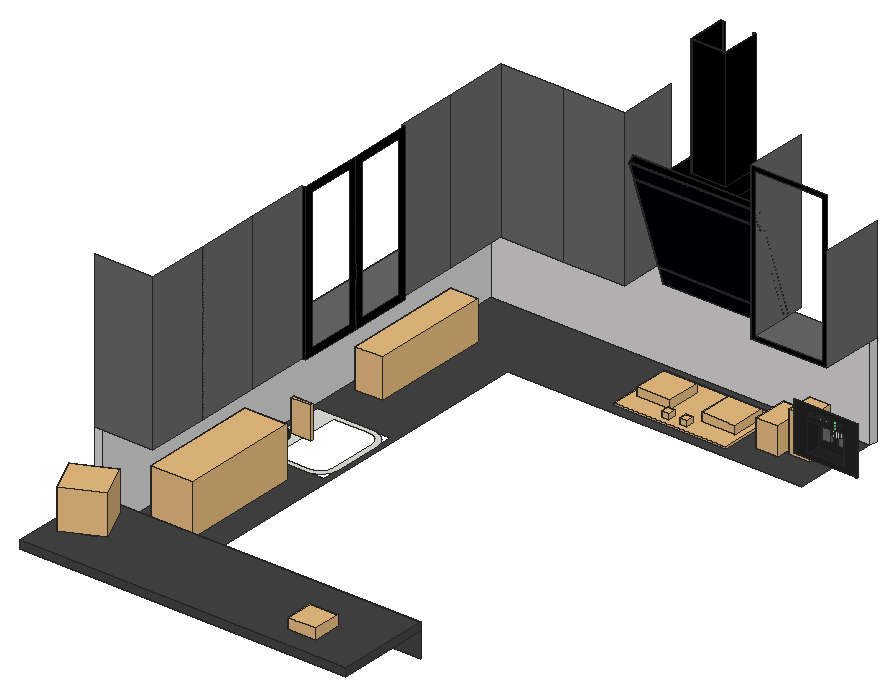
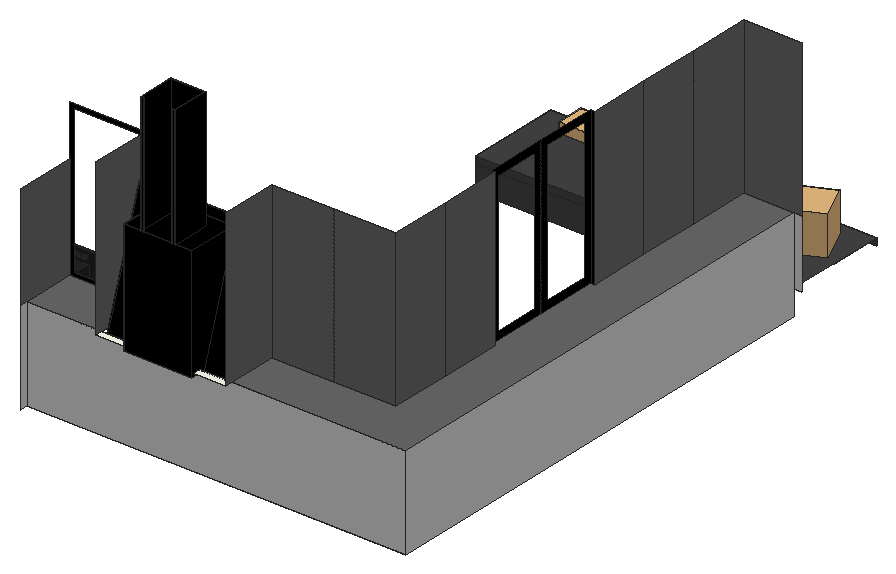
# SketchUp Ruby script. Lengths in inches.
U = 1.inch
M = Sketchup.active_model
def pt(a) = Geom::Point3d.new(a.map { |v| v * U })
def face(e, loops, mat)
  f = e.add_face(loops[0].map { |a| pt(a) })
  loops[1..].each { |l| e.add_face(l.map { |a| pt(a) }).erase! }
  f.material = f.back_material = mat if mat
  f
end
# faces: each face lists its corners as indices into pts; further lists are holes
def faces(e, pts, list, mat = nil) = list.each { |f| face(e, (f[0].is_a?(Array) ? f : [f]).map { |l| l.map { |i| pts[i] } }, mat) }
# xy, xz, yz: faces in a plane at the given z, y or x. An outline is a flat list of corners, or four numbers for a rectangle; further outlines are holes
def ring(l) = l.size == 4 ? [[l[0], l[1]], [l[2], l[1]], [l[2], l[3]], [l[0], l[3]]] : l.each_slice(2).to_a
def flat(e, list, mat, &to3) = list.each { |f| face(e, (f[0].is_a?(Array) ? f : [f]).map { |l| ring(l).map { |u, v| to3.(u, v) } }, mat) }
def xy(e, z, list, mat = nil) = flat(e, list, mat) { |x, y| [x, y, z] }
def xz(e, y, list, mat = nil) = flat(e, list, mat) { |x, z| [x, y, z] }
def yz(e, x, list, mat = nil) = flat(e, list, mat) { |y, z| [x, y, z] }
def lines(e, pts, list) = list.each { |a, b| e.add_line(pt(pts[a]), pt(pts[b])) }
# prism: a flat outline (further loops are holes) pulled along v
def prism(e, loops, v, mat = nil)
  f = face(e, loops, mat); d = Geom::Vector3d.new(v.map { |x| x * U })
  f.pushpull(f.normal.samedirection?(d) ? d.length : -d.length)
end
def box(e, o, s, mat = nil) = prism(e, [[o, [o[0] + s[0], o[1], o[2]], [o[0] + s[0], o[1] + s[1], o[2]], [o[0], o[1] + s[1], o[2]]]], [0, 0, s[2]], mat)
def at(x, y, z, deg = 0) = Geom::Transformation.translation(pt([x, y, z])) * Geom::Transformation.rotation(ORIGIN, Z_AXIS, deg.degrees)
def axes(o, x, y, z) = Geom::Transformation.new([*x, 0, *y, 0, *z, 0, *pt(o).to_a, 1])
def part(name) = M.definitions.add(name)
# library, detail: a bought-in or finely detailed component or shape, given as its bounding box
def library(name, o, s) = part(name).tap { |d| box(d.entities, o, s) }
def detail(e, o, s) = box(e.add_group.entities, o, s)
def put(e, d, t, mat = nil) = e.add_instance(d, t).tap { |i| i.material = mat if mat }
def group(e, t, mat = nil) = e.add_group.tap { |g| g.transformation = t; g.material = mat if mat }.entities
root = M.entities
M.materials.add("78970012").color = [84, 74, 27]
M.materials.add("Brush Stainles Steel").color = [21, 26, 31]
M.materials.add("Material60").color = [0, 0, 8]
M.materials.add("[0046_Gold]").color = [255, 215, 0]
M.materials.add("[0053_Ivory]").color = [255, 255, 240]
M.materials.add("[0067_PaleGreen]").color = [152, 251, 152]
M.materials.add("[0070_SpringGreen]").color = [0, 255, 127]
M.materials.add("[0072_DarkSeaGreen]").color = [143, 188, 143]
M.materials.add("[0087_Cyan]").color = [0, 255, 255]
M.materials.add("[0088_Aquamarine]").color = [127, 255, 212]
M.materials.add("[0096_SkyBlue]").color = [135, 206, 235]
M.materials.add("[0117_GhostWhite]").color = [248, 248, 255]
M.materials.add("[0131_Silver]").color = [192, 192, 192]
M.materials.add("[0134_DimGray]").color = [105, 105, 105]
M.materials.add("[0136_Charcoal]").color = [35, 35, 35]
M.materials.add("[0137_Black]").color = [0, 0, 0]
M.materials.add("[Granite Dark Gray]").color = [69, 68, 68]
M.materials.add("[Stone Vein Gray]").color = [219, 217, 217]
M.materials.add("stainless-steel2").color = [0, 0, 0]
c1 = library("Group70\#2",[-9.87,-9.87,-55.07],[19.74,112.51,110.23])
c2 = library("组\#1",[0,0,0],[5.3125,6.7,10.38])
c3 = library("Gas burner",[0,0.01,0],[8.66,8.66,2.72])
c4 = part("Bathroom Tap Knob")
xy(c4.entities,1.57,[[0.59,0,0.74,0.02,0.89,0.08,1.01,0.17,1.1,0.3,1.16,0.4375,1.18,0.59,1.16,0.74,1.1,0.89,1.01,1.01,0.89,1.1,0.74,1.16,0.59,1.18,0.4375,1.16,0.3,1.1,0.17,1.01,0.08,0.89,0.02,0.74,0,0.59,0.02,0.4375,0.08,0.3,0.17,0.17,0.3,0.08,0.4375,0.02]])
p = [[0.3,0.08,0],[0.4375,0.02,0],[0.4375,0.02,1.57],[0.3,0.08,1.57],[0.59,0,0],[0.59,0,1.57],
  [0.74,0.02,0],[0.74,0.02,1.57],[0.89,0.08,0],[0.89,0.08,1.57],[0.17,0.17,0],[0.17,0.17,1.57],
  [1.01,0.17,0],[1.01,0.17,1.57],[0.08,0.3,0],[0.08,0.3,1.57],[1.1,0.3,0],[1.1,0.3,1.57],
  [0.02,0.4375,0],[0.02,0.4375,1.57],[1.16,0.4375,0],[1.16,0.4375,1.57],[0,0.59,0],[0,0.59,1.57],
  [1.18,0.59,0],[1.18,0.59,1.57],[0.02,0.74,0],[0.02,0.74,1.57],[1.16,0.74,0],[1.16,0.74,1.57],
  [0.08,0.89,0],[0.08,0.89,1.57],[1.1,0.89,0],[1.1,0.89,1.57],[0.17,1.01,0],[0.17,1.01,1.57],
  [1.01,1.01,0],[1.01,1.01,1.57],[0.3,1.1,0],[0.3,1.1,1.57],[0.89,1.1,0],[0.89,1.1,1.57],
  [0.4375,1.16,0],[0.4375,1.16,1.57],[0.74,1.16,0],[0.74,1.16,1.57],[0.59,1.18,0],[0.59,1.18,1.57]]
faces(c4.entities,p,[[0,1,2,3],[1,4,5,2],[4,6,7,5],[6,8,9,7],[10,0,3,11],[8,12,13,9],[14,10,11,15],[12,16,17,13],
  [18,14,15,19],[16,20,21,17],[22,18,19,23],[20,24,25,21],[26,22,23,27],[24,28,29,25],[30,26,27,31],[28,32,33,29],
  [34,30,31,35],[32,36,37,33],[38,34,35,39],[36,40,41,37],[42,38,39,43],[40,44,45,41],[46,42,43,47],[44,46,47,45]])
c5 = library("Bathroom Tap",[0,0,0],[4.72,0.79,8.27])
c6 = library("Group\#260",[0,0,0],[30.82,7.02,10])
c7 = library("GasStove_E",[0,-1.18,0],[28.74,16.53,0.59])
c8 = library("knifes set",[0,0,0],[30.4,10.88,12.79])
c9 = library("Group71\#2",[-14.38,-9.9375,-11.98],[31.13,19.875,24.75])
c10 = library("Burner control knob",[0,0,0],[1.95,1.95,1.42])
c11 = part("KNIFE\#1")
p = [[0,0.99,0.32],[0,0.99,0.35]]
lines(c11.entities,p,[[0,1]])
c12 = library("Group39\#2",[-175.75,-175.61,-127.36],[351.08,350.86,254.72])
c13 = library("Group40\#2",[-253.94,153.82,-285.05],[511.41,519.67,535.99])
c14 = library("Group49\#3",[-60.66,-60.66,-22.72],[121.32,121.32,45.44])
c15 = part("Group38\#2")
xy(c15.entities,0,[[-16.45,-149.33,16.45,-149.33,48.64,-142.8,78.71,-130.03,105.33,-111.58,127.35,-88.26,143.81,-61.07,153.98,-31.22,157.42,0,153.98,31.22,143.81,61.07,127.35,88.26,105.33,111.58,78.71,130.03,48.64,142.8,16.45,149.33,-16.45,149.33,-48.64,142.8,-78.71,130.03,-105.33,111.58,-127.35,88.26,-143.81,61.07,-153.98,31.22,-157.42,0,-153.98,-31.22,-143.81,-61.07,-127.35,-88.26,-105.33,-111.58,-78.71,-130.03,-48.64,-142.8]],"78970012")
c16 = library("Light",[0.01,0,0],[0.32,0.16,0.01])
c17 = library("Up\#1",[0.01,0,0],[0.17,0.15,0.01])
c18 = library("Deep Freeze",[0.01,0,0],[0.81,0.15,0.01])
c19 = library("Temp: 0*",[0.02,0,0],[0.98,0.22,0.01])
c20 = library("Down",[0.01,0,0],[0.36,0.12,0.01])
c21 = library("Crushed Ice",[0.01,0,0],[0.77,0.13,0.01])
c22 = part("komin dół\#1")
prism(c22.entities,[[[9.06,9.76,0],[9.06,9.84,0],[9.92,9.84,0],[9.92,-0.08,0],[-0.08,-0.08,0],[-0.08,9.84,0],[0.79,9.84,0],[0.79,9.76,0],[0.08,9.76,0],[0.08,0.08,0],[9.76,0.08,0],[9.76,9.76,0]]],[0,0,18.125],"stainless-steel2")
c23 = part("komin")
put(c23.entities,c22,at(0,0,0),"Brush Stainles Steel")
c24 = part("korpus")
prism(c24.entities,[[[0,0,17.125],[0,13.78,17.125],[0,13.78,0],[0,9.89,0]]],[19.69,0,0],"stainless-steel2")
c25 = part("panel przód")
yz(c25.entities,0,[[11.02,0,9.65,2.39,9.82,2.49,11.19,0.1],[9.45,2.73,1.57,16.37,1.75,16.47,2.63,14.93,8.34,5.04,8.73,4.36,9.62,2.83],[1.38,16.71,0,19.09,0.17,19.19,1.55,16.81]],"Material60")
yz(c25.entities,0,[[11.19,0.1,9.82,2.49,9.99,2.58,8.9,4.46,8.73,4.36,8.34,5.04,2.63,14.93,2.8,15.03,1.72,16.9,1.55,16.81,0.17,19.19,1.19,19.78,12.22,0.6875]],"stainless-steel2")
yz(c25.entities,35.43,[[11.02,0,11.19,0.1,9.82,2.49,9.65,2.39],[9.45,2.73,9.62,2.83,8.73,4.36,8.34,5.04,2.63,14.93,1.75,16.47,1.57,16.37],[1.38,16.71,1.55,16.81,0.17,19.19,0,19.09]],"Material60")
yz(c25.entities,35.43,[[11.19,0.1,12.22,0.6875,1.19,19.78,0.17,19.19,1.55,16.81,1.72,16.9,2.8,15.03,2.63,14.93,8.34,5.04,8.73,4.36,8.9,4.46,9.99,2.58,9.82,2.49]],"stainless-steel2")
p = [[0,9.65,2.39],[0,11.02,0],[35.43,11.02,0],[35.43,9.65,2.39],[0,11.19,0.1],[35.43,11.19,0.1],
  [0,9.82,2.49],[35.43,9.82,2.49],[0,12.22,0.6875],[35.43,12.22,0.6875],[0,1.19,19.78],[35.43,1.19,19.78],
  [0,9.99,2.58],[35.43,9.99,2.58],[0,8.9,4.46],[35.43,8.9,4.46],[0,1.57,16.37],[0,9.45,2.73],
  [35.43,9.45,2.73],[35.43,1.57,16.37],[0,9.62,2.83],[35.43,9.62,2.83],[0,8.73,4.36],[35.43,8.73,4.36],
  [0,8.34,5.04],[35.43,8.34,5.04],[0,2.63,14.93],[35.43,2.63,14.93],[0,1.75,16.47],[35.43,1.75,16.47],
  [0,2.8,15.03],[35.43,2.8,15.03],[0,1.72,16.9],[35.43,1.72,16.9],[0,0,19.09],[0,1.38,16.71],
  [35.43,1.38,16.71],[35.43,0,19.09],[0,1.55,16.81],[35.43,1.55,16.81],[0,0.17,19.19],[35.43,0.17,19.19]]
faces(c25.entities,p,[[0,1,2,3],[1,4,5,2],[4,6,7,5],[6,0,3,7],[16,17,18,19],[17,20,21,18],[20,22,23,21],[22,24,25,23],
  [24,26,27,25],[26,28,29,27],[28,16,19,29],[34,35,36,37],[35,38,39,36],[38,40,41,39],[40,34,37,41]],"Material60")
faces(c25.entities,p,[[4,8,9,5],[8,10,11,9],[12,6,7,13],[14,12,13,15],[22,14,15,23],[30,26,27,31],[32,30,31,33],[38,32,33,39],
  [10,40,41,11]],"stainless-steel2")
c26 = part("BERG Spring 90")
p = [[27.56,1.88,18.59],[27.56,1.19,19.78]]
lines(c26.entities,p,[[0,1]])
put(c26.entities,c23,at(12.8,5.82,18.59))
put(c26.entities,c24,at(7.875,1.88,1.46))
put(c26.entities,c25,at(0,0,0))
c27 = library("Hold Temperature",[0.01,0,0],[1.21,0.16,0.01])
c28 = library("Temp: 37*",[0.02,0,0],[1.12,0.22,0.01])
c29 = library("Up",[0.01,0,0],[0.17,0.15,0.01])
c30 = library("Cubed Ice",[0.01,0,0],[0.63,0.13,0.01])
c31 = library("Down\#1",[0.01,0,0],[0.36,0.12,0.01])
xy(root,42,[[[8.58,105.62,22.51,105.62,23.18,105.66,23.83,105.78,24.45,105.98,25.05,106.25,25.6,106.59,26.1,107,26.53,107.47,26.9,107.98,27.19,108.53,27.41,109.12,27.54,109.72,27.58,110.34,27.58,122.55,27.54,123.16,27.41,123.77,27.19,124.35,26.9,124.91,26.53,125.42,26.1,125.89,25.6,126.29,25.05,126.64,24.45,126.91,23.83,127.11,23.18,127.23,22.51,127.27,8.58,127.27],[13.65,106.8,13.65,126.09,22.47,126.09,23.01,126.06,23.5,125.97,23.97,125.82,24.41,125.61,24.83,125.35,25.2,125.05,25.53,124.7,25.8,124.32,26.02,123.9,26.18,123.46,26.28,123.01,26.3125,122.51,26.3125,110.38,26.28,109.88,26.18,109.42,26.02,108.99,25.8,108.57,25.53,108.1875,25.2,107.84,24.83,107.53,24.41,107.27,23.97,107.07,23.5,106.92,23.01,106.83,22.47,106.8],[11.11,116.05,11,116.0625,10.9,116.1,10.82,116.17,10.75,116.25,10.71,116.34,10.69,116.44,10.71,116.55,10.75,116.64,10.82,116.72,10.9,116.78,11,116.82,11.11,116.84,11.22,116.82,11.32,116.78,11.41,116.72,11.48,116.64,11.52,116.55,11.54,116.44,11.52,116.34,11.48,116.25,11.41,116.17,11.32,116.1,11.22,116.0625]],[11.11,116.05,11.22,116.0625,11.32,116.1,11.41,116.17,11.48,116.25,11.52,116.34,11.54,116.44,11.52,116.55,11.48,116.64,11.41,116.72,11.32,116.78,11.22,116.82,11.11,116.84,11,116.82,10.9,116.78,10.82,116.72,10.75,116.64,10.71,116.55,10.69,116.44,10.71,116.34,10.75,116.25,10.82,116.17,10.9,116.1,11,116.0625]])
xy(root,42,[[[7,59.91,29,59.91,29,163,104.87,163,104.87,185,7,185],[8.58,105.62,27.58,127.27]]],"[Granite Dark Gray]")
xy(root,48.49,[[7,35.93,7,46.93,8.78,46.93,8.78,47.93,10.56,47.93,10.56,46.93,12.33,46.93,12.33,47.93,14.11,47.93,14.11,46.93,15.89,46.93,15.89,47.93,17.67,47.93,17.67,46.93,19.44,46.93,19.44,47.93,21.22,47.93,21.22,46.93,23,46.93,23,47.93,24.78,47.93,24.78,46.93,26.56,46.93,26.56,47.93,28.33,47.93,28.33,46.93,30.11,46.93,30.11,47.93,31.89,47.93,31.89,46.93,33.67,46.93,33.67,47.93,35.44,47.93,35.44,46.93,37.22,46.93,37.22,47.93,39,47.93,39,46.93,40.78,46.93,40.78,47.93,42.56,47.93,42.56,46.93,44.33,46.93,44.33,47.93,46.11,47.93,46.11,46.93,47.89,46.93,47.89,47.93,49.67,47.93,49.67,46.93,51.44,46.93,51.44,47.93,53.22,47.93,53.22,46.93,55,46.93,55,47.93,56.78,47.93,56.78,46.93,58.56,46.93,58.56,47.93,60.33,47.93,60.33,46.93,62.11,46.93,62.11,47.93,63.89,47.93,63.89,46.93,65.67,46.93,65.67,47.93,67.44,47.93,67.44,46.93,69.22,46.93,69.22,47.93,71,47.93,71,46.93,72.78,46.93,72.78,47.93,74.56,47.93,74.56,46.93,76.33,46.93,76.33,47.93,78.11,47.93,78.11,46.93,79.89,46.93,79.89,47.93,81.67,47.93,81.67,46.93,83.44,46.93,83.44,47.93,85.22,47.93,85.22,46.93,87,46.93,87,35.93]],"[Granite Dark Gray]")
xy(root,50.49,[[5,35.93,89,59.93]],"[Granite Dark Gray]")
xy(root,52.26,[[106.25,158.7,122.66,158.94]])
xy(root,53.6,[[109.84,158.7,119.07,161.85]],"[0136_Charcoal]")
xy(root,56.05,[[111.39,161.36,113.77,161.85],[115.39,161.36,117.72,161.85]],"[0134_DimGray]")
xy(root,59.04,[[111.39,161.36,113.77,161.85]],"[0134_DimGray]")
xy(root,59.11,[[115.39,161.36,117.72,161.85]],"[0131_Silver]")
xy(root,59.35,[[[116.49,158.95,116.14,159.01,115.8125,159.16,115.54,159.38,115.33,159.67,115.2,160,115.17,160.35,115.24,160.6875,115.39,161.01,115.62,161.27,115.91,161.47,116.25,161.59,116.61,161.625,116.97,161.5625,117.29,161.42,117.57,161.19,117.78,160.91,117.9,160.58,117.93,160.23,117.87,159.89,117.72,159.57,117.49,159.3,117.19,159.1,116.85,158.98],[116.5,159.11,116.82,159.13,117.12,159.24,117.38,159.42,117.58,159.65,117.72,159.93,117.77,160.24,117.75,160.54,117.64,160.83,117.45,161.09,117.21,161.29,116.92,161.42,116.61,161.47,116.29,161.44,115.99,161.34,115.73,161.16,115.52,160.92,115.39,160.64,115.33,160.34,115.36,160.03,115.47,159.74,115.65,159.49,115.9,159.29,116.1875,159.16]]])
xy(root,60.19,[[[112.5625,160.53,112.5,160.54,112.4375,160.56,112.39,160.6,112.35,160.65,112.32,160.71,112.3125,160.77,112.32,160.83,112.35,160.89,112.39,160.94,112.4375,160.98,112.5,161,112.5625,161.01,112.63,161,112.6875,160.98,112.74,160.94,112.78,160.89,112.8,160.83,112.8125,160.77,112.8,160.71,112.78,160.65,112.74,160.6,112.6875,160.56,112.63,160.54],[112.5625,160.6,112.61,160.61,112.65,160.625,112.68,160.65,112.71,160.6875,112.73,160.73,112.73,160.8125,112.71,160.85,112.68,160.89,112.65,160.91,112.61,160.93,112.5625,160.9375,112.52,160.93,112.44,160.89,112.41,160.85,112.4,160.8125,112.39,160.77,112.4,160.73,112.41,160.6875,112.44,160.65,112.48,160.625,112.52,160.61]]])
xy(root,61.17,[[116.5,159.11,116.1875,159.16,115.9,159.29,115.65,159.49,115.47,159.74,115.36,160.03,115.33,160.34,115.39,160.64,115.52,160.92,115.73,161.16,115.99,161.34,116.29,161.44,116.61,161.47,116.92,161.42,117.21,161.29,117.45,161.09,117.64,160.83,117.75,160.54,117.77,160.24,117.72,159.93,117.58,159.65,117.38,159.42,117.12,159.24,116.82,159.13],[112.5625,160.6,112.52,160.61,112.48,160.625,112.44,160.65,112.41,160.6875,112.4,160.73,112.39,160.77,112.4,160.8125,112.41,160.85,112.44,160.89,112.52,160.93,112.5625,160.9375,112.61,160.93,112.65,160.91,112.68,160.89,112.71,160.85,112.73,160.8125,112.73,160.73,112.71,160.6875,112.68,160.65,112.65,160.625,112.61,160.61]])
xy(root,61.17,[[[109.84,158.7,119.07,161.85],[116.49,158.95,116.85,158.98,117.19,159.1,117.49,159.3,117.72,159.57,117.87,159.89,117.93,160.23,117.9,160.58,117.78,160.91,117.57,161.19,117.29,161.42,116.97,161.5625,116.61,161.625,116.25,161.59,115.91,161.47,115.62,161.27,115.39,161.01,115.24,160.6875,115.17,160.35,115.2,160,115.33,159.67,115.54,159.38,115.8125,159.16,116.14,159.01],[112.5625,160.53,112.63,160.54,112.6875,160.56,112.74,160.6,112.78,160.65,112.8,160.71,112.8125,160.77,112.8,160.83,112.78,160.89,112.74,160.94,112.6875,160.98,112.63,161,112.5625,161.01,112.5,161,112.4375,160.98,112.39,160.94,112.35,160.89,112.32,160.83,112.3125,160.77,112.32,160.71,112.35,160.65,112.39,160.6,112.4375,160.56,112.5,160.54]]],"[0136_Charcoal]")
xy(root,64.76,[[106.25,158.7,122.66,158.94]])
xy(root,66,[[52,185,85.34,187]],"[0053_Ivory]")
xy(root,66,[[7,60,7,185,52,185,52,172,20,172,20,140,21,140,21,108,20,108,20,60],[85.34,171,104.87,185]],"[0134_DimGray]")
xz(root,35.93,[[5,48.49,89,50.49]],"[Granite Dark Gray]")
xz(root,59.93,[[5,48.49,7,50.49]],"[0053_Ivory]")
xz(root,59.93,[[7,48.49,89,50.49]],"[Granite Dark Gray]")
xz(root,60,[[5,66,20,106]],"[0134_DimGray]")
xz(root,108,[[20,66,21,106]],"[0137_Black]")
xz(root,140,[[20,66,21,106]],"[0137_Black]")
xz(root,158.7,[[115.29,62.08,115.35,62.08,115.42,62.09,115.47,62.12,115.52,62.16,115.56,62.22,115.58,62.28,115.58,62.35,115.57,62.41,115.54,62.47,115.5,62.52,115.44,62.55,115.38,62.57,115.3125,62.58,115.25,62.5625,115.19,62.53,115.14,62.49,115.11,62.4375,115.09,62.375,115.08,62.31,115.1,62.25,115.125,62.1875,115.17,62.14,115.22,62.1],[112.32,62.15,112.38,62.16,112.44,62.18,112.5,62.22,112.53,62.27,112.56,62.33,112.57,62.4,112.56,62.46,112.5,62.58,112.38,62.64,112.32,62.65,112.25,62.64,112.19,62.61,112.14,62.58,112.1,62.52,112.08,62.46,112.07,62.4,112.08,62.33,112.1,62.27,112.14,62.22,112.19,62.18,112.25,62.16],[115.32,62.81,115.39,62.82,115.45,62.84,115.5,62.88,115.54,62.93,115.5625,62.99,115.57,63.06,115.5625,63.12,115.54,63.18,115.5,63.23,115.45,63.27,115.39,63.3,115.32,63.31,115.26,63.3,115.2,63.27,115.14,63.23,115.11,63.18,115.08,63.12,115.07,63.06,115.08,62.99,115.11,62.93,115.14,62.88,115.2,62.84,115.26,62.82],[112.32,62.83,112.38,62.84,112.44,62.86,112.5,62.9,112.53,62.95,112.56,63.01,112.57,63.08,112.56,63.14,112.5,63.26,112.44,63.3,112.38,63.32,112.32,63.33,112.25,63.32,112.19,63.3,112.14,63.26,112.1,63.2,112.08,63.14,112.07,63.08,112.08,63.01,112.1,62.95,112.14,62.9,112.19,62.86,112.25,62.84]],"[0046_Gold]")
xz(root,158.7,[[116.63,62.74,117.1875,63.3]],"[0067_PaleGreen]")
xz(root,158.7,[[116.63,62.06,117.1875,62.61]],"[0070_SpringGreen]")
xz(root,158.7,[[116.63,61.36,117.1875,61.92]],"[0072_DarkSeaGreen]")
xz(root,158.7,[[110.36,62.15,110.42,62.16,110.48,62.18,110.53,62.22,110.57,62.27,110.6,62.33,110.61,62.4,110.6,62.46,110.57,62.52,110.53,62.58,110.48,62.61,110.42,62.64,110.36,62.65,110.29,62.64,110.23,62.61,110.18,62.58,110.14,62.52,110.12,62.46,110.11,62.4,110.12,62.33,110.14,62.27,110.18,62.22,110.23,62.18,110.29,62.16]],"[0087_Cyan]")
xz(root,158.7,[[110.35,62.83,110.42,62.84,110.48,62.86,110.53,62.9,110.57,62.95,110.6,63.01,110.61,63.08,110.6,63.14,110.58,63.2,110.54,63.25,110.49,63.29,110.43,63.32,110.36,63.33,110.3,63.32,110.24,63.3,110.18,63.26,110.14,63.21,110.12,63.15,110.11,63.08,110.11,63.02,110.14,62.96,110.18,62.9,110.23,62.86,110.29,62.84]],"[0088_Aquamarine]")
xz(root,158.7,[[112.82,62.15,114.82,62.63],[112.83,62.82,114.83,63.3]],"[0096_SkyBlue]")
xz(root,158.7,[[[106.25,52.26,122.66,64.76],[109.84,53.6,119.07,61.17],[112.83,62.82,114.83,63.3],[112.82,62.15,114.82,62.63],[116.63,62.74,117.1875,63.3],[116.63,62.06,117.1875,62.61],[116.63,61.36,117.1875,61.92],[115.32,62.81,115.26,62.82,115.2,62.84,115.14,62.88,115.11,62.93,115.08,62.99,115.07,63.06,115.08,63.12,115.11,63.18,115.14,63.23,115.2,63.27,115.26,63.3,115.32,63.31,115.39,63.3,115.45,63.27,115.5,63.23,115.54,63.18,115.5625,63.12,115.57,63.06,115.5625,62.99,115.54,62.93,115.5,62.88,115.45,62.84,115.39,62.82],[110.36,62.15,110.29,62.16,110.23,62.18,110.18,62.22,110.14,62.27,110.12,62.33,110.11,62.4,110.12,62.46,110.14,62.52,110.18,62.58,110.23,62.61,110.29,62.64,110.36,62.65,110.42,62.64,110.48,62.61,110.53,62.58,110.57,62.52,110.6,62.46,110.61,62.4,110.6,62.33,110.57,62.27,110.53,62.22,110.48,62.18,110.42,62.16],[110.35,62.83,110.29,62.84,110.23,62.86,110.18,62.9,110.14,62.96,110.11,63.02,110.11,63.08,110.12,63.15,110.14,63.21,110.18,63.26,110.24,63.3,110.3,63.32,110.36,63.33,110.43,63.32,110.49,63.29,110.54,63.25,110.58,63.2,110.6,63.14,110.61,63.08,110.6,63.01,110.57,62.95,110.53,62.9,110.48,62.86,110.42,62.84],[112.32,62.15,112.25,62.16,112.19,62.18,112.14,62.22,112.1,62.27,112.08,62.33,112.07,62.4,112.08,62.46,112.1,62.52,112.14,62.58,112.19,62.61,112.25,62.64,112.32,62.65,112.38,62.64,112.5,62.58,112.56,62.46,112.57,62.4,112.56,62.33,112.53,62.27,112.5,62.22,112.44,62.18,112.38,62.16],[112.32,62.83,112.25,62.84,112.19,62.86,112.14,62.9,112.1,62.95,112.08,63.01,112.07,63.08,112.08,63.14,112.1,63.2,112.14,63.26,112.19,63.3,112.25,63.32,112.32,63.33,112.38,63.32,112.44,63.3,112.5,63.26,112.56,63.14,112.57,63.08,112.56,63.01,112.53,62.95,112.5,62.9,112.44,62.86,112.38,62.84],[115.29,62.08,115.22,62.1,115.17,62.14,115.125,62.1875,115.1,62.25,115.08,62.31,115.09,62.375,115.11,62.4375,115.14,62.49,115.19,62.53,115.25,62.5625,115.3125,62.58,115.38,62.57,115.44,62.55,115.5,62.52,115.54,62.47,115.57,62.41,115.58,62.35,115.58,62.28,115.56,62.22,115.52,62.16,115.47,62.12,115.42,62.09,115.35,62.08]]],"[0136_Charcoal]")
xz(root,161.36,[[111.39,56.05,113.77,59.04],[115.39,56.05,117.72,59.11]],"[0134_DimGray]")
xz(root,161.85,[[[109.84,53.6,119.07,61.17],[115.39,56.05,117.72,59.11],[111.39,56.05,113.77,59.04]]],"[0136_Charcoal]")
xz(root,171,[[[85.34,66,104.87,106],[86.34,67,103.87,105]]],"[0137_Black]")
xz(root,172,[[20,66,36,106],[36,66,52,106]],"[0134_DimGray]")
xz(root,185,[[7,42,104.87,66]],"[Stone Vein Gray]")
yz(root,7,[[59.91,42,185,42,185,66,60,66,59.93,48.49]],"[Stone Vein Gray]")
yz(root,20,[[60,66,76,106],[76,66,92,106],[92,66,108,106],[140,66,156,106],[156,66,172,106]],"[0134_DimGray]")
yz(root,21,[[[108,66,124,106],[110,68,122,104]],[[124,66,140,106],[126,68,138,104]]],"[0137_Black]")
yz(root,52,[[172,66,187,106]],"[0134_DimGray]")
yz(root,85.34,[[171,66,187,106]],"[0134_DimGray]")
yz(root,89,[[35.93,48.49,59.93,50.49]],"[Granite Dark Gray]")
yz(root,104.87,[[171,66,187,92.99]],"[0134_DimGray]")
yz(root,104.87,[[185,42,187,66]],"[Stone Vein Gray]")
yz(root,106.25,[[158.7,52.26,158.94,64.76]])
yz(root,109.84,[[158.7,53.6,161.85,61.17]],"[0136_Charcoal]")
yz(root,111.39,[[161.36,56.05,161.85,59.04]],"[0134_DimGray]")
yz(root,112.73,[[160.73,60.19,160.77,61.17],[160.77,60.19,160.8125,61.17]])
yz(root,113.77,[[161.36,56.05,161.85,59.04]],"[0134_DimGray]")
yz(root,115.39,[[161.36,56.05,161.85,59.11]],"[0134_DimGray]")
yz(root,117.72,[[161.36,56.05,161.85,59.11]],"[0134_DimGray]")
yz(root,119.07,[[158.7,53.6,161.85,61.17]],"[0136_Charcoal]")
yz(root,122.66,[[158.7,52.26,158.94,64.76]])
p = [[7,59.91,42],[7,59.93,48.49],[89,59.93,48.49],[89,59.91,42],[29,59.91,42],[5,59.93,48.49],
  [7,60,66],[5,60,66],[116.14,159.01,61.17],[115.8125,159.16,61.17],[115.8125,159.16,59.35],[116.14,159.01,59.35],
  [116.49,158.95,61.17],[116.49,158.95,59.35],[116.85,158.98,61.17],[116.85,158.98,59.35],[117.19,159.1,61.17],[117.19,159.1,59.35],
  [116.1875,159.16,61.17],[116.5,159.11,61.17],[116.5,159.11,59.35],[116.1875,159.16,59.35],[116.82,159.13,61.17],[116.82,159.13,59.35],
  [117.12,159.24,61.17],[117.12,159.24,59.35],[117.49,159.3,61.17],[117.49,159.3,59.35],[115.54,159.38,61.17],[115.54,159.38,59.35],
  [115.9,159.29,61.17],[115.9,159.29,59.35],[117.38,159.42,61.17],[117.38,159.42,59.35],[115.65,159.49,61.17],[115.65,159.49,59.35],
  [117.72,159.57,61.17],[117.72,159.57,59.35],[115.33,159.67,61.17],[115.33,159.67,59.35],[117.58,159.65,61.17],[117.58,159.65,59.35],
  [115.47,159.74,61.17],[115.47,159.74,59.35],[117.87,159.89,61.17],[117.87,159.89,59.35],[115.2,160,61.17],[115.2,160,59.35],
  [115.36,160.03,61.17],[115.36,160.03,59.35],[117.72,159.93,61.17],[117.72,159.93,59.35],[117.77,160.24,61.17],[117.77,160.24,59.35],
  [117.93,160.23,61.17],[117.93,160.23,59.35],[115.17,160.35,61.17],[115.17,160.35,59.35],[115.33,160.34,61.17],[115.33,160.34,59.35],
  [117.75,160.54,61.17],[117.75,160.54,59.35],[117.9,160.58,61.17],[117.9,160.58,59.35],[115.24,160.6875,61.17],[115.24,160.6875,59.35],
  [115.39,160.64,61.17],[115.39,160.64,59.35],[117.64,160.83,61.17],[117.64,160.83,59.35],[115.52,160.92,61.17],[115.52,160.92,59.35],
  [117.78,160.91,61.17],[117.78,160.91,59.35],[115.39,161.01,61.17],[115.39,161.01,59.35],[117.45,161.09,61.17],[117.45,161.09,59.35],
  [115.73,161.16,61.17],[115.73,161.16,59.35],[117.57,161.19,61.17],[117.57,161.19,59.35],[115.62,161.27,61.17],[115.62,161.27,59.35],
  [117.21,161.29,61.17],[117.21,161.29,59.35],[115.99,161.34,61.17],[115.99,161.34,59.35],[117.29,161.42,61.17],[117.29,161.42,59.35],
  [115.91,161.47,61.17],[115.91,161.47,59.35],[116.29,161.44,61.17],[116.29,161.44,59.35],[116.92,161.42,61.17],[116.92,161.42,59.35],
  [116.61,161.47,61.17],[116.61,161.47,59.35],[116.97,161.5625,61.17],[116.97,161.5625,59.35],[116.25,161.59,61.17],[116.25,161.59,59.35],
  [116.61,161.625,61.17],[116.61,161.625,59.35],[112.5,160.54,61.17],[112.4375,160.56,61.17],[112.4375,160.56,60.19],[112.5,160.54,60.19],
  [112.5625,160.53,61.17],[112.5625,160.53,60.19],[112.6875,160.56,61.17],[112.63,160.54,61.17],[112.63,160.54,60.19],[112.6875,160.56,60.19],
  [112.39,160.6,61.17],[112.35,160.65,61.17],[112.35,160.65,60.19],[112.39,160.6,60.19],[112.32,160.71,61.17],[112.32,160.71,60.19],
  [112.44,160.65,61.17],[112.48,160.625,61.17],[112.48,160.625,60.19],[112.44,160.65,60.19],[112.52,160.61,61.17],[112.5625,160.6,61.17],
  [112.5625,160.6,60.19],[112.52,160.61,60.19],[112.61,160.61,61.17],[112.61,160.61,60.19],[112.65,160.625,61.17],[112.65,160.625,60.19],
  [112.68,160.65,61.17],[112.68,160.65,60.19],[112.78,160.65,61.17],[112.74,160.6,61.17],[112.74,160.6,60.19],[112.78,160.65,60.19],
  [112.8,160.71,61.17],[112.8,160.71,60.19],[112.3125,160.77,61.17],[112.3125,160.77,60.19],[112.39,160.77,61.17],[112.4,160.73,61.17],
  [112.4,160.73,60.19],[112.39,160.77,60.19],[112.41,160.6875,61.17],[112.41,160.6875,60.19],[112.71,160.6875,61.17],[112.71,160.6875,60.19],
  [112.73,160.73,61.17],[112.73,160.73,60.19],[112.8125,160.77,61.17],[112.8125,160.77,60.19],[112.32,160.83,61.17],[112.32,160.83,60.19],
  [112.35,160.89,61.17],[112.35,160.89,60.19],[112.41,160.85,61.17],[112.4,160.8125,61.17],[112.4,160.8125,60.19],[112.41,160.85,60.19],
  [112.73,160.8125,61.17],[112.71,160.85,61.17],[112.71,160.85,60.19],[112.73,160.8125,60.19],[112.78,160.89,61.17],[112.8,160.83,61.17],
  [112.8,160.83,60.19],[112.78,160.89,60.19],[112.39,160.94,61.17],[112.39,160.94,60.19],[112.4375,160.98,61.17],[112.4375,160.98,60.19],
  [112.48,160.91,61.17],[112.44,160.89,61.17],[112.44,160.89,60.19],[112.48,160.91,60.19],[112.5625,160.9375,61.17],[112.52,160.93,61.17],
  [112.52,160.93,60.19],[112.5625,160.9375,60.19],[112.68,160.89,61.17],[112.65,160.91,61.17],[112.65,160.91,60.19],[112.68,160.89,60.19],
  [112.61,160.93,61.17],[112.61,160.93,60.19],[112.6875,160.98,61.17],[112.74,160.94,61.17],[112.74,160.94,60.19],[112.6875,160.98,60.19],
  [112.5,161,61.17],[112.5,161,60.19],[112.5625,161.01,61.17],[112.5625,161.01,60.19],[112.63,161,61.17],[112.63,161,60.19],
  [23.18,105.66,42],[27.58,105.62,42]]
faces(root,p,[[0,1,2,3,4]],"[Granite Dark Gray]")
faces(root,p,[[5,1,6,7]],"[Stone Vein Gray]")
faces(root,p,[[8,9,10,11],[12,8,11,13],[14,12,13,15],[16,14,15,17],[18,19,20,21],[19,22,23,20],[22,24,25,23],[26,16,17,27],
  [9,28,29,10],[30,18,21,31],[24,32,33,25],[34,30,31,35],[36,26,27,37],[28,38,39,29],[32,40,41,33],[42,34,35,43],
  [44,36,37,45],[38,46,47,39],[48,42,43,49],[40,50,51,41],[50,52,53,51],[54,44,45,55],[46,56,57,47],[58,48,49,59],
  [52,60,61,53],[62,54,55,63],[56,64,65,57],[66,58,59,67],[60,68,69,61],[70,66,67,71],[72,62,63,73],[64,74,75,65],
  [68,76,77,69],[78,70,71,79],[80,72,73,81],[74,82,83,75],[76,84,85,77],[86,78,79,87],[88,80,81,89],[82,90,91,83],
  [92,86,87,93],[84,94,95,85],[96,92,93,97],[94,96,97,95],[98,88,89,99],[90,100,101,91],[100,102,103,101],[102,98,99,103],
  [104,105,106,107],[108,104,107,109],[110,111,112,113],[111,108,109,112],[114,115,116,117],[115,118,119,116],[105,114,117,106],[120,121,122,123],
  [124,125,126,127],[121,124,127,122],[125,128,129,126],[128,130,131,129],[130,132,133,131],[134,135,136,137],[135,110,113,136],[138,134,137,139],
  [118,140,141,119],[142,143,144,145],[143,146,147,144],[146,120,123,147],[132,148,149,133],[148,150,151,149],[152,138,139,153],[140,154,155,141],
  [154,156,157,155],[158,159,160,161],[159,142,145,160],[162,163,164,165],[166,167,168,169],[167,152,153,168],[156,170,171,157],[170,172,173,171],
  [174,175,176,177],[175,158,161,176],[178,179,180,181],[179,174,177,180],[182,183,184,185],[183,186,187,184],[186,178,181,187],[188,189,190,191],
  [189,166,169,190],[163,182,185,164],[172,192,193,173],[192,194,195,193],[194,196,197,195],[196,188,191,197]])
lines(root,p,[[198,199]])
put(root,c1,axes([89.09,172.84,42.39],[0,0,-0.04196],[0.04184,-0.00315,0],[0.00315,0.04184,0]))
put(root,c2,at(94.39,171.92,42))
put(root,c3,at(56.16,170.62,42))
put(root,c3,at(72.89,170.62,42))
put(root,c4,axes([10.48,113.56,42],[1.07244,0,0],[0,1,0],[0,0,1]))
put(root,c4,axes([10.48,118.48,42],[1.07244,0,0],[0,1,0],[0,0,1]))
put(root,c5,axes([10.69,116.05,42],[1.07244,0,0],[0,1,0],[0,0,1]))
put(root,c6,at(16.63,138.09,42,90))
put(root,c7,at(54.48,166.67,42.12))
put(root,c8,at(22.47,69.65,42.43,90))
put(root,c9,axes([91.21,172.9,46.08],[0,0.28124,0],[0.28124,0,0],[0,0,0.28124]))
put(root,c10,at(67.46,166.92,42.71,90))
put(root,c10,at(72.1875,166.88,42.71,90))
put(root,c11,axes([-0.76,84.38,47.64],[0,-0.01461,0.99989],[-1,0,0],[0,-0.99989,-0.01461]))
put(root,c12,axes([13.22,47.92,52.17],[0.01216,0.00443,0],[0.00443,-0.01216,0],[0,0,0.01294]))
put(root,c13,axes([12.94,48.39,48.96],[-0.00829,0.01779,0],[0,0,0.01963],[0.01779,0.00829,0]))
put(root,c14,axes([75.79,41.73,53.9],[0,0.05842,0],[0.05842,0,0],[0,0,0.05842]))
put(root,c15,axes([13.23,54.53,53.5],[0.01216,0.00443,0],[0.00443,-0.01216,0],[0,0,0.01294]))
put(root,c16,axes([117.75,158.7,61.53],[1,0,0],[0,0,1],[0,-0.9675,0]))
put(root,c17,axes([115.25,158.7,62.25],[1,0,0],[0,0,1],[0,-0.9675,0]),"[0046_Gold]")
put(root,c18,axes([117.54,158.7,62.25],[1,0,0],[0,0,1],[0,-0.9675,0]))
put(root,c19,axes([113.33,158.7,62.29],[1,0,0],[0,0,1],[0,-0.9675,0]))
put(root,c20,axes([112.14,158.7,62.3125],[1,0,0],[0,0,1],[0,-0.9675,0]))
put(root,c21,axes([110.84,158.7,62.32],[1,0,0],[0,0,1],[0,-0.9675,0]))
put(root,c26,axes([53.36,171.76,62.39],[0.90257,0,0],[0,0.97787,0],[0,0,1.71128]))
put(root,c27,axes([117.41,158.7,62.95],[1,0,0],[0,0,1],[0,-0.9675,0]))
put(root,c28,axes([113.28,158.7,62.95],[1,0,0],[0,0,1],[0,-0.9675,0]))
put(root,c29,axes([115.23,158.7,62.99],[1,0,0],[0,0,1],[0,-0.9675,0]))
put(root,c30,axes([110.82,158.7,63.03],[1,0,0],[0,0,1],[0,-0.9675,0]),"[0117_GhostWhite]")
put(root,c31,axes([112.14,158.7,63.04],[1,0,0],[0,0,1],[0,-0.9675,0]))
